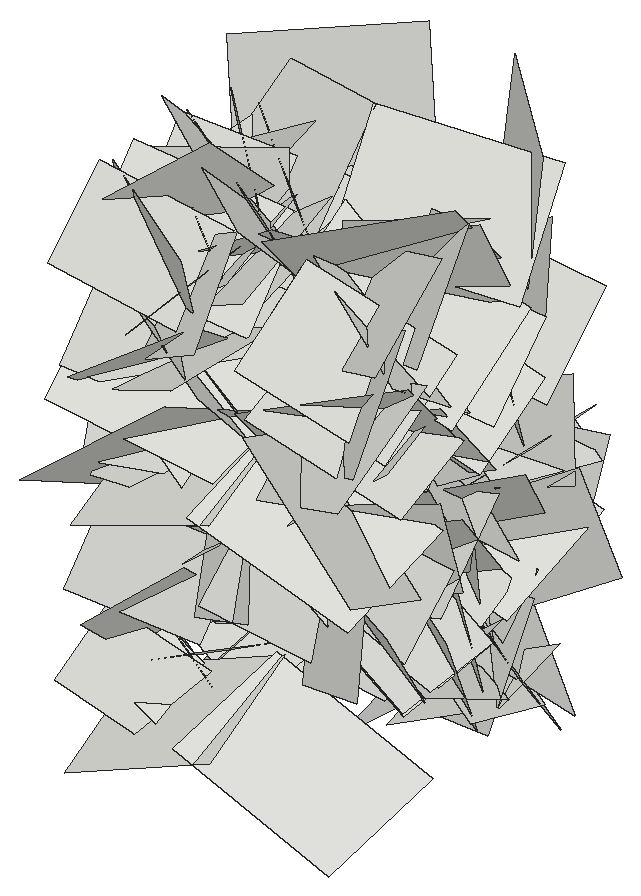
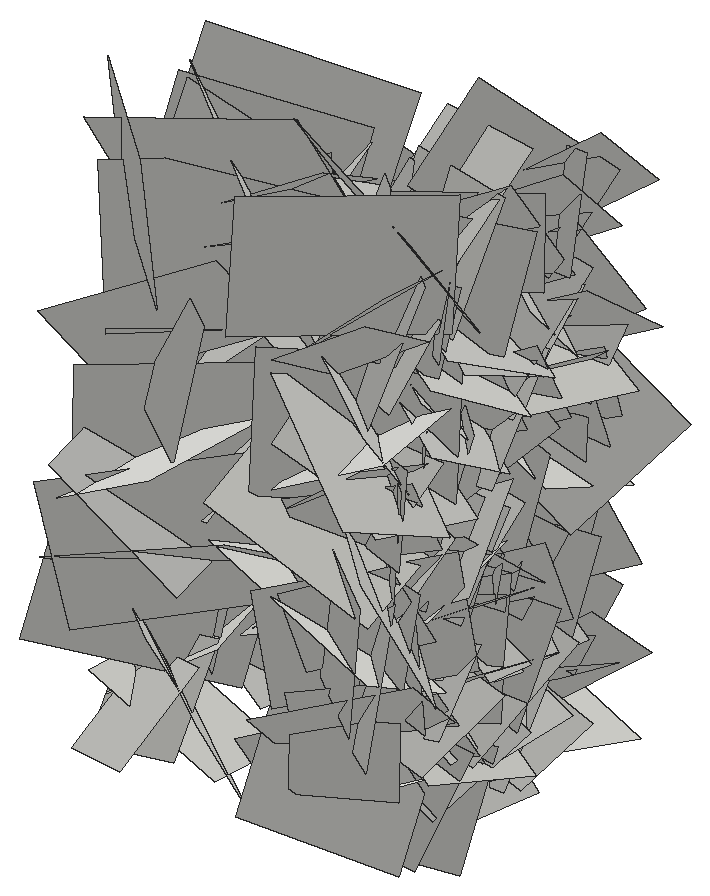
# SketchUp Ruby script. Lengths in inches.
U = 1.inch
M = Sketchup.active_model
def pt(a) = Geom::Point3d.new(a.map { |v| v * U })
def face(e, loops, mat)
  f = e.add_face(loops[0].map { |a| pt(a) })
  loops[1..].each { |l| e.add_face(l.map { |a| pt(a) }).erase! }
  f.material = f.back_material = mat if mat
  f
end
# faces: each face lists its corners as indices into pts; further lists are holes
def faces(e, pts, list, mat = nil) = list.each { |f| face(e, (f[0].is_a?(Array) ? f : [f]).map { |l| l.map { |i| pts[i] } }, mat) }
# xy, xz, yz: faces in a plane at the given z, y or x. An outline is a flat list of corners, or four numbers for a rectangle; further outlines are holes
def ring(l) = l.size == 4 ? [[l[0], l[1]], [l[2], l[1]], [l[2], l[3]], [l[0], l[3]]] : l.each_slice(2).to_a
def flat(e, list, mat, &to3) = list.each { |f| face(e, (f[0].is_a?(Array) ? f : [f]).map { |l| ring(l).map { |u, v| to3.(u, v) } }, mat) }
def xy(e, z, list, mat = nil) = flat(e, list, mat) { |x, y| [x, y, z] }
def xz(e, y, list, mat = nil) = flat(e, list, mat) { |x, z| [x, y, z] }
def yz(e, x, list, mat = nil) = flat(e, list, mat) { |y, z| [x, y, z] }
def lines(e, pts, list) = list.each { |a, b| e.add_line(pt(pts[a]), pt(pts[b])) }
# prism: a flat outline (further loops are holes) pulled along v
def prism(e, loops, v, mat = nil)
  f = face(e, loops, mat); d = Geom::Vector3d.new(v.map { |x| x * U })
  f.pushpull(f.normal.samedirection?(d) ? d.length : -d.length)
end
def box(e, o, s, mat = nil) = prism(e, [[o, [o[0] + s[0], o[1], o[2]], [o[0] + s[0], o[1] + s[1], o[2]], [o[0], o[1] + s[1], o[2]]]], [0, 0, s[2]], mat)
def at(x, y, z, deg = 0) = Geom::Transformation.translation(pt([x, y, z])) * Geom::Transformation.rotation(ORIGIN, Z_AXIS, deg.degrees)
def axes(o, x, y, z) = Geom::Transformation.new([*x, 0, *y, 0, *z, 0, *pt(o).to_a, 1])
def part(name) = M.definitions.add(name)
# library, detail: a bought-in or finely detailed component or shape, given as its bounding box
def library(name, o, s) = part(name).tap { |d| box(d.entities, o, s) }
def detail(e, o, s) = box(e.add_group.entities, o, s)
def put(e, d, t, mat = nil) = e.add_instance(d, t).tap { |i| i.material = mat if mat }
def group(e, t, mat = nil) = e.add_group.tap { |g| g.transformation = t; g.material = mat if mat }.entities
root = M.entities
c1 = part("Component\#6")
p = [[0.01,0,0],[0,3.24,4.54],[4.32,3.24,4.54],[4.33,0,0]]
faces(c1.entities,p,[[0,1,2,3]])
put(root,c1,axes([28.31,163.43,17.5],[0.07736,-0.30856,0.98844],[0.18729,0.98007,0.2929],[-1.08152,0.14765,0.12143]))
put(root,c1,axes([24.34,163.43,17.5],[-0.07736,-0.30856,0.98844],[-0.18729,0.98007,0.2929],[1.08152,0.14765,0.12143]))
put(root,c1,axes([24.34,155.625,2.89],[0.13104,0.56412,0.5606],[-0.11872,0.57403,-0.55293],[0.83462,-0.00692,-0.16667]))
put(root,c1,axes([24.34,168.54,15.47],[-0.051,0.16682,-0.79913],[0.09039,-0.79511,-0.17112],[0.86061,0.0934,-0.02938]))
put(root,c1,axes([28.31,164.44,22.83],[0.02931,-0.02413,-0.88007],[0.04764,-0.87932,0.02552],[-0.93201,-0.0457,-0.02637]))
put(root,c1,axes([24.34,159.9,13.67],[-0.02397,0.44215,0.82689],[-0.11898,0.8199,-0.44149],[0.98679,0.1096,-0.03314]))
put(root,c1,axes([24.34,159.79,6],[-0.13547,0.51146,0.93772],[-0.15367,0.92736,-0.52557],[1.12174,0.18881,0.04125]))
put(root,c1,axes([28.31,165.07,9.38],[-0.13081,0.27606,-0.70722],[0.08788,-0.70731,-0.29057],[-0.79993,-0.12284,0.08373]))
put(root,c1,axes([24.34,167.39,19.82],[0.12929,0.6108,0.35138],[0.02449,0.35295,-0.62154],[0.74654,-0.11736,-0.04046]))
put(root,c1,axes([24.34,155.24,20.59],[0.01301,0.69003,0.71111],[-0.211,0.69839,-0.67424],[1.02891,0.13449,-0.14726]))
put(root,c1,axes([24.34,164.66,7.18],[-0.03191,0.54978,-0.59147],[0.106,-0.58478,-0.54866],[0.84939,0.09364,0.04625]))
put(root,c1,axes([24.34,167.84,10.46],[-0.01526,0.23241,-0.73689],[0.14958,-0.72384,-0.23105],[0.80526,0.13886,0.02896]))
put(root,c1,axes([24.34,166.25,3.34],[0.10377,-0.78092,-0.09398],[-0.04515,-0.09983,0.78516],[0.83253,0.09192,0.05429]))
put(root,c1,axes([24.34,166.67,11.65],[0.03639,0.32382,0.70516],[0.0632,0.70266,-0.32558],[0.82009,-0.06852,-0.0062]))
put(root,c1,axes([28.31,164.7,6.68],[0.19863,-0.78204,0.62344],[0.03401,0.63866,0.7915],[-1.0596,-0.1261,0.14227]))
put(root,c1,axes([28.31,165.06,16.01],[0.24936,0.99659,0.4051],[0.07669,0.39908,-1.02378],[-1.13774,0.24532,0.01978]))
put(root,c1,axes([28.31,162.4,12.14],[-0.15913,-0.1111,0.71617],[0.10617,0.72117,0.13287],[-0.76084,0.12387,-0.13124]))
put(root,c1,axes([24.34,166.02,4.84],[-0.16866,0.71959,0.68076],[0.0323,0.69272,-0.72511],[1.04952,0.09433,0.13172]))
put(root,c1,axes([24.34,157.37,3.29],[0.12325,0.67494,0.21472],[0.06797,0.20667,-0.68436],[0.74769,-0.13004,0.02682]))
put(root,c1,axes([24.34,162.54,0.74],[-0.05881,-0.79857,0.25436],[0.14334,0.24305,0.79255],[0.87675,-0.0933,-0.11251]))
put(root,c1,axes([24.34,164.04,2.37],[-0.08884,-0.86849,0.07962],[0.14736,0.06566,0.86256],[0.91264,-0.09515,-0.13152]))
put(root,c1,axes([28.31,167.12,21.5],[-0.0656,0.35319,-0.61189],[-0.00255,-0.61434,-0.35436],[-0.7489,-0.02885,0.0548]))
put(root,c1,axes([28.31,165.55,15.88],[0.02597,-0.35934,-0.67832],[-0.02345,-0.67872,0.35875],[-0.81334,0.00809,-0.032]))
put(root,c1,axes([28.31,169.26,18.83],[-0.02849,-0.83115,-0.05333],[0.13283,-0.05679,0.82186],[-0.87278,0.01849,0.12683]))
put(root,c1,axes([24.34,168.08,9.41],[-0.11593,0.02752,-0.90523],[0.14705,-0.90054,-0.04413],[0.94866,0.14295,-0.10378]))
put(root,c1,axes([28.31,161.46,7.67],[-0.11157,-0.00104,0.59962],[-0.09459,0.60203,-0.01462],[-0.62852,-0.09042,-0.10424]))
put(root,c1,axes([28.31,169.83,13.22],[-0.13817,-0.64015,-0.16037],[0.03989,-0.17041,0.64965],[-0.69839,0.11692,0.06883]))
put(root,c1,axes([24.34,170.98,12.21],[-0.31631,-0.51758,-1.19288],[-0.16648,-1.20059,0.56021],[1.36826,-0.26573,-0.20761]))
put(root,c1,axes([28.31,164.04,15.7],[-0.03624,-0.6234,-0.24842],[-0.08,-0.24359,0.62167],[-0.70683,0.05954,-0.05762]))
put(root,c1,axes([28.31,160.57,3.12],[-0.03509,0.82869,0.13415],[0.15764,0.13792,-0.81528],[-0.87577,-0.00838,-0.15213]))
put(root,c1,axes([24.34,159.03,23.29],[-0.13252,0.38295,-0.87838],[0.10893,-0.87536,-0.39626],[1.00987,0.14467,-0.07253]))
put(root,c1,axes([28.31,166.8,6.58],[0.19077,-0.84984,-0.315],[-0.00737,-0.32244,0.86593],[-0.9607,-0.16629,-0.0692]))
put(root,c1,axes([24.34,166.22,16.78],[-0.0558,0.90138,-0.08554],[0.09664,-0.07998,-0.89882],[0.95488,0.06076,0.08597]))
put(root,c1,axes([28.31,169.73,5.36],[-0.07377,0.11031,-0.61615],[-0.06228,-0.61836,-0.10407],[-0.66058,0.04598,0.07863]))
put(root,c1,axes([28.31,159.32,12.84],[-0.06752,-0.16321,-0.59207],[-0.0871,-0.58763,0.17083],[-0.64514,0.09641,0.0389]))
put(root,c1,axes([24.34,167.39,3.05],[-0.22625,-1.02118,-0.283],[0.12014,-0.30902,1.02962],[1.11681,-0.17363,-0.16809]))
put(root,c1,axes([28.31,159.79,25.07],[0.1328,0.69586,-0.68383],[0.18687,-0.69425,-0.67416],[-1.01714,-0.03669,-0.21313]))
put(root,c1,axes([24.34,163.26,10.51],[0.09772,0.8385,-0.3881],[-0.10419,-0.37892,-0.842],[0.97385,-0.12468,-0.05114]))
put(root,c1,axes([28.31,160.97,6.7],[-0.04912,0.73058,0.10133],[0.09877,0.10652,-0.72536],[-0.77557,-0.03271,-0.0988]))
put(root,c1,axes([24.34,170.16,13.55],[-0.14984,-1.04824,-0.22204],[0.00627,-0.22472,1.05715],[1.13577,-0.13705,-0.03513]))
put(root,c1,axes([28.31,161.26,10.83],[0.08958,0.45503,-0.59155],[-0.06652,-0.58889,-0.46195],[-0.78829,0.10141,-0.02824]))
put(root,c1,axes([28.31,160.54,14.42],[0.065,-0.29459,-0.75204],[0.0763,-0.74921,0.29935],[-0.85274,-0.0895,-0.03054]))
put(root,c1,axes([28.31,160.65,18.69],[-0.1336,-0.1743,0.59472],[0.06624,0.60023,0.18916],[-0.65357,0.09646,-0.1024]))
put(root,c1,axes([28.31,159.61,12.59],[-0.0897,0.16152,-0.57424],[-0.01993,-0.58042,-0.16049],[-0.632,-0.00462,0.08656]))
put(root,c1,axes([24.34,169.09,13.37],[0.12805,-0.81492,0.2825],[-0.01832,0.28292,0.8235],[0.91406,0.11983,-0.02307]))
put(root,c1,axes([28.31,158.82,19.64],[-0.09205,0.73549,-0.019],[0.17536,0.00088,-0.72213],[-0.75991,-0.08889,-0.16434]))
put(root,c1,axes([24.34,166.72,20.27],[0.14718,0.45385,-0.66356],[0.05291,-0.67695,-0.45256],[0.85051,-0.03642,0.14299]))
put(root,c1,axes([24.34,158.84,13.7],[0.15038,-0.75335,0.50607],[-0.08727,0.49942,0.76653],[0.95804,0.16374,-0.00961]))
put(root,c1,axes([24.34,161.03,4.22],[0.00206,0.54706,-0.73945],[0.10036,-0.73565,-0.544],[0.96983,0.07497,0.05787]))
put(root,c1,axes([24.34,167.74,3.51],[-0.11337,-0.86322,0.3774],[0.28126,0.33685,0.84566],[0.95821,-0.201,-0.20357]))
put(root,c1,axes([24.34,165.75,-1.09],[-0.03685,-0.4153,0.96157],[-0.02645,0.96216,0.41465],[1.10996,0.00914,0.04181]))
put(root,c1,axes([24.34,165.51,17.74],[0.00528,-0.97827,-0.44464],[-0.11526,-0.44282,0.97306],[1.13321,-0.04048,0.10104]))
put(root,c1,axes([28.31,158.25,7.85],[-0.01053,0.60228,-0.51533],[0.19634,-0.49934,-0.58716],[-0.81696,-0.12777,-0.13447]))
put(root,c1,axes([28.31,167.39,12.19],[0.06725,0.11282,-0.6237],[-0.12717,-0.61335,-0.12315],[-0.65971,0.12973,-0.03984]))
put(root,c1,axes([28.31,164.71,11.17],[0.09162,-0.23701,0.75882],[0.09076,0.76162,0.22813],[-0.83777,0.05659,0.1077]))
put(root,c1,axes([24.34,164.72,6.23],[-0.02586,0.29335,1.1723],[-0.23754,1.1511,-0.29271],[1.25874,0.22326,-0.03115]))
put(root,c1,axes([28.31,159.82,10.86],[0.164,0.05549,-0.7166],[-0.119,-0.72215,-0.08015],[-0.75252,0.12629,-0.14349]))
put(root,c1,axes([24.34,167.01,8.33],[0.18631,0.3359,0.73427],[0.04897,0.74605,-0.35235],[0.8545,-0.11599,-0.1399]))
put(root,c1,axes([24.34,166.18,19.56],[-0.12535,0.0531,1.28965],[-0.2192,1.27754,-0.07157],[1.35051,0.21229,0.10808]))
put(root,c1,axes([24.34,168.14,0.12],[-0.06773,-0.63363,0.78179],[0.11595,0.77435,0.63654],[1.06038,-0.12515,-0.01967]))
put(root,c1,axes([24.34,169.19,10.7],[-0.0913,0.46499,-1.24639],[-0.29576,-1.22753,-0.43867],[1.37875,-0.23253,-0.17663]))
put(root,c1,axes([28.31,165.96,10.85],[0.09912,0.20412,-0.70693],[0.02587,-0.71308,-0.20267],[-0.77953,0.00229,-0.09661]))
put(root,c1,axes([28.31,161.25,17.66],[0.25985,0.898,-0.37026],[0.14737,-0.41038,-0.90325],[-1.01902,0.16964,-0.22504]))
put(root,c1,axes([28.31,162.79,15.86],[0.07285,0.46729,0.4905],[-0.02436,0.49435,-0.46773],[-0.71769,0.03066,0.06566]))
put(root,c1,axes([24.34,167.22,15.375],[-0.0235,-0.92066,-0.53568],[-0.01768,-0.53543,0.92093],[1.12894,-0.02755,0.00327]))
put(root,c1,axes([24.34,167.28,17.92],[-0.19972,-0.96368,-0.57877],[0.14667,-0.60226,0.95775],[1.18251,-0.08806,-0.21655]))
put(root,c1,axes([24.34,157.18,19.73],[-0.07599,0.81527,0.8297],[-0.084,0.82592,-0.8184],[1.23014,0.10676,-0.00463]))
put(root,c1,axes([24.34,167.18,1.59],[-0.07507,-1.0991,0.32301],[-0.05871,0.32653,1.09895],[1.2129,-0.05222,0.07319]))
put(root,c1,axes([24.34,168.87,14.79],[0.03205,0.06087,-1.12787],[-0.16204,-1.11767,-0.06442],[1.18627,-0.15431,0.02167]))
put(root,c1,axes([24.34,166.01,11.8],[0.21466,0.53877,-0.68228],[-0.03009,-0.69607,-0.55809],[0.92102,-0.14831,0.14079]))
put(root,c1,axes([24.34,163.57,3.71],[0.11292,-0.2033,0.99476],[-0.09749,0.99417,0.21302],[1.07181,0.11185,-0.08542]))
put(root,c1,axes([24.34,159.91,9.22],[-0.2022,-1.20502,0.50539],[-0.1049,0.52261,1.20871],[1.38114,-0.13672,0.1658]))
put(root,c1,axes([24.34,162.44,14.8125],[-0.22172,-1.13603,-0.19278],[0.19013,-0.22565,1.13507],[1.20652,-0.17321,-0.21429]))
put(root,c1,axes([24.34,160.62,5.12],[0.08568,1.04485,0.18773],[-0.09569,0.19436,-1.04286],[1.1212,-0.06325,-0.10335]))
put(root,c1,axes([28.31,162.91,7.6875],[0.03517,0.6334,0.29771],[0.1292,0.28826,-0.62688],[-0.73053,0.08147,-0.09654]))
put(root,c1,axes([24.34,163.93,5.47],[0.11462,-1.01834,-0.26907],[-0.10191,-0.2789,1.0169],[1.11183,0.07941,0.12095]))
put(root,c1,axes([24.34,156.14,6.5],[0.17845,0.35117,0.84391],[0.01887,0.85668,-0.36003],[0.96872,-0.08137,-0.14844]))
put(root,c1,axes([28.31,170.02,6.34],[0.13634,-0.30577,-0.6303],[0.02329,-0.63876,0.31436],[-0.74222,-0.07621,-0.10592]))
put(root,c1,axes([24.34,160.14,4.78],[0.03826,-0.47304,0.81506],[0.18962,0.80427,0.45886],[0.98077,-0.13704,-0.12051]))
put(root,c1,axes([24.34,166.625,12.7],[0.17127,1.04033,-0.10676],[-0.13463,-0.08771,-1.04688],[1.10034,-0.17266,-0.11147]))
put(root,c1,axes([24.34,168.99,0.33],[0.20008,-0.71049,0.66963],[-0.07161,0.67089,0.73087],[1.03242,0.18422,-0.07908]))
put(root,c1,axes([24.34,164.18,5.53],[0.00871,-1.21515,-0.1589],[-0.11926,-0.15898,1.20995],[1.29354,-0.00648,0.11262]))
put(root,c1,axes([28.31,159.77,13.93],[0.14822,0.47929,0.38572],[-0.01533,0.39801,-0.48932],[-0.65196,0.0996,0.0992]))
put(root,c1,axes([24.34,165.6875,8.33],[0.14254,-0.77018,0.64298],[0.05856,0.65343,0.77114],[1.06187,0.06735,-0.12884]))
put(root,c1,axes([24.34,164.53,2.65],[0.11418,0.95876,0.15487],[0.16789,0.13639,-0.95453],[1.01568,-0.13033,0.14037]))
put(root,c1,axes([24.34,170.79,17.67],[0.07972,-0.69903,-0.88266],[-0.01234,-0.88506,0.69994],[1.19343,0.03754,0.0662]))
put(root,c1,axes([24.34,165.97,13.03],[0.11695,-0.23373,1.15092],[-0.10796,1.14973,0.24325],[1.24018,0.12213,-0.08736]))
put(root,c1,axes([28.31,164.09,3.1],[0.16189,-0.51758,0.36968],[0.06161,0.38995,0.52196],[-0.67139,-0.08902,0.13704]))
put(root,c1,axes([24.34,155.93,16.01],[0.06166,0.77521,1.08886],[-0.24821,1.07895,-0.75564],[1.39492,0.15772,-0.18259]))
put(root,c1,axes([24.34,163.21,2.24],[-0.08398,-0.53221,1.10764],[0.11648,1.10243,0.53756],[1.29738,-0.13342,0.02343]))
put(root,c1,axes([24.34,161.02,12.77],[0.04866,0.36936,-1.04237],[0.12613,-1.03886,-0.36288],[1.16543,0.09701,0.0828]))
put(root,c1,axes([24.34,162.03,18.62],[0.15865,-0.78055,-0.79386],[-0.03617,-0.80384,0.78393],[1.17956,0.08034,0.13081]))
put(root,c1,axes([24.34,161.03,16.77],[-0.02327,0.73455,-0.90907],[0.17416,-0.89826,-0.72978],[1.22657,0.14148,0.08637]))
put(root,c1,axes([24.34,163.86,1.73],[0.03729,0.66749,1.03354],[-0.00972,1.03407,-0.66752],[1.30413,-0.01138,-0.03452]))
put(root,c1,axes([24.34,162.85,15.75],[0.04254,-1.00522,0.67204],[0.02385,0.67292,1.00519],[1.28151,0.02084,-0.04102]))
put(root,c1,axes([24.34,163.36,23.49],[0.04873,0.57368,-1.00395],[0.12423,-1.00188,-0.56714],[1.21936,0.07915,0.09791]))
put(root,c1,axes([24.34,159.69,18.96],[0.02704,0.74145,1.09535],[-0.09362,1.09406,-0.73853],[1.39894,0.05888,-0.07059]))
put(root,c1,axes([24.34,166.4,18.65],[-0.092,-1.19571,-0.63762],[0.0325,-0.6405,1.19693],[1.43603,-0.06211,-0.06794]))
put(root,c1,axes([24.34,155.03,14.95],[-0.10989,1.07322,0.82249],[0.07177,0.82799,-1.07186],[1.43147,0.04087,0.11688]))
put(root,c1,axes([24.34,159.14,18.38],[0.07521,0.79304,-0.86536],[0.12573,-0.86735,-0.78513],[1.23784,0.03991,0.13233]))
put(root,c1,axes([24.34,168.375,23.9],[-0.0952,-0.72561,-1.04974],[0.29336,-1.03837,0.69407],[1.32049,0.17837,-0.22987]))
put(root,c1,axes([24.34,157.93,15.34],[0.27083,1.19165,0.15594],[-0.0802,0.17506,-1.21378],[1.27139,-0.2428,-0.10978]))
put(root,c1,axes([24.34,162.31,11.53],[0.17206,0.75955,-0.87532],[0.12131,-0.89005,-0.75111],[1.22246,-0.01858,0.19774]))
put(root,c1,axes([24.34,165.1,2.71],[-0.06092,-1.21711,0.58199],[0.18306,0.57109,1.21136],[1.41828,-0.12599,-0.13136]))
put(root,c1,axes([24.34,170.58,10.37],[0.24309,-1.14649,0.14454],[0.04952,0.15643,1.16674],[1.2239,0.22139,-0.07591]))
put(root,c1,axes([24.34,161.07,7.88],[0.0926,0.91308,0.78861],[0.24837,0.76278,-0.90913],[1.25453,-0.21841,0.12178]))
put(root,c1,axes([24.34,171.01,11.29],[0.23144,-0.15428,-1.27652],[-0.01824,-1.29503,0.15357],[1.36284,0.00887,0.21884]))
put(root,c1,axes([24.34,167.61,21.95],[0.32344,0.31012,-1.26322],[-0.1451,-1.28265,-0.34796],[1.37111,-0.2089,0.26116]))
put(root,c1,axes([24.34,161.91,24.73],[0.20116,0.87735,-0.9177],[0.06395,-0.93308,-0.87958],[1.34427,-0.0869,0.17917]))
put(root,c1,axes([24.34,161.24,11.55],[0.08722,-1.18104,-0.51149],[0.30261,-0.48302,1.16122],[1.33028,0.18731,-0.23062]))
put(root,c1,axes([24.34,160.65,1.35],[0.1594,-1.22011,-0.46707],[0.28659,-0.43091,1.2127],[1.35486,0.2347,-0.20157]))
put(root,c1,axes([24.34,170.67,8.29],[0.13658,-1.14766,-0.62909],[0.33753,-0.58565,1.13362],[1.34561,0.26339,-0.2205]))
put(root,c1,axes([24.34,161.87,9.58],[0.35888,-0.49511,-1.17449],[0.11741,-1.19919,0.53746],[1.34594,0.23663,0.26628]))
put(root,c1,axes([38.11,161.87,9.58],[-0.35888,-0.49511,-1.17449],[-0.11741,-1.19919,0.53746],[-1.34594,0.23663,0.26628]))
put(root,c1,axes([38.11,170.67,8.29],[-0.13658,-1.14766,-0.62909],[-0.33753,-0.58565,1.13362],[-1.34561,0.26339,-0.2205]))
put(root,c1,axes([38.11,160.65,1.35],[-0.1594,-1.22011,-0.46707],[-0.28659,-0.43091,1.2127],[-1.35486,0.2347,-0.20157]))
put(root,c1,axes([38.11,161.24,11.55],[-0.08722,-1.18104,-0.51149],[-0.30261,-0.48302,1.16122],[-1.33028,0.18731,-0.23062]))
put(root,c1,axes([38.11,161.91,24.73],[-0.20116,0.87735,-0.9177],[-0.06395,-0.93308,-0.87958],[-1.34427,-0.0869,0.17917]))
put(root,c1,axes([38.11,167.61,21.95],[-0.32344,0.31012,-1.26322],[0.1451,-1.28265,-0.34796],[-1.37111,-0.2089,0.26116]))
put(root,c1,axes([38.11,171.01,11.29],[-0.23144,-0.15428,-1.27652],[0.01824,-1.29503,0.15357],[-1.36284,0.00887,0.21884]))
put(root,c1,axes([38.11,161.07,7.88],[-0.0926,0.91308,0.78861],[-0.24837,0.76278,-0.90913],[-1.25453,-0.21841,0.12178]))
put(root,c1,axes([38.11,170.58,10.37],[-0.24309,-1.14649,0.14454],[-0.04952,0.15643,1.16674],[-1.2239,0.22139,-0.07591]))
put(root,c1,axes([38.11,165.1,2.71],[0.06092,-1.21711,0.58199],[-0.18306,0.57109,1.21136],[-1.41828,-0.12599,-0.13136]))
put(root,c1,axes([38.11,162.31,11.53],[-0.17206,0.75955,-0.87532],[-0.12131,-0.89005,-0.75111],[-1.22246,-0.01858,0.19774]))
put(root,c1,axes([38.11,157.93,15.34],[-0.27083,1.19165,0.15594],[0.0802,0.17506,-1.21378],[-1.27139,-0.2428,-0.10978]))
put(root,c1,axes([38.11,168.375,23.9],[0.0952,-0.72561,-1.04974],[-0.29336,-1.03837,0.69407],[-1.32049,0.17837,-0.22987]))
put(root,c1,axes([38.11,159.14,18.38],[-0.07521,0.79304,-0.86536],[-0.12573,-0.86735,-0.78513],[-1.23784,0.03991,0.13233]))
put(root,c1,axes([38.11,155.03,14.95],[0.10989,1.07322,0.82249],[-0.07177,0.82799,-1.07186],[-1.43147,0.04087,0.11688]))
put(root,c1,axes([38.11,166.4,18.65],[0.092,-1.19571,-0.63762],[-0.0325,-0.6405,1.19693],[-1.43603,-0.06211,-0.06794]))
put(root,c1,axes([38.11,159.69,18.96],[-0.02704,0.74145,1.09535],[0.09362,1.09406,-0.73853],[-1.39894,0.05888,-0.07059]))
put(root,c1,axes([38.11,163.36,23.49],[-0.04873,0.57368,-1.00395],[-0.12423,-1.00188,-0.56714],[-1.21936,0.07915,0.09791]))
put(root,c1,axes([38.11,162.85,15.75],[-0.04254,-1.00522,0.67204],[-0.02385,0.67292,1.00519],[-1.28151,0.02084,-0.04102]))
put(root,c1,axes([38.11,163.86,1.73],[-0.03729,0.66749,1.03354],[0.00972,1.03407,-0.66752],[-1.30413,-0.01138,-0.03452]))
put(root,c1,axes([38.11,161.03,16.77],[0.02327,0.73455,-0.90907],[-0.17416,-0.89826,-0.72978],[-1.22657,0.14148,0.08637]))
put(root,c1,axes([38.11,162.03,18.62],[-0.15865,-0.78055,-0.79386],[0.03617,-0.80384,0.78393],[-1.17956,0.08034,0.13081]))
put(root,c1,axes([38.11,161.02,12.77],[-0.04866,0.36936,-1.04237],[-0.12613,-1.03886,-0.36288],[-1.16543,0.09701,0.0828]))
put(root,c1,axes([38.11,163.21,2.24],[0.08398,-0.53221,1.10764],[-0.11648,1.10243,0.53756],[-1.29738,-0.13342,0.02343]))
put(root,c1,axes([38.11,155.93,16.01],[-0.06166,0.77521,1.08886],[0.24821,1.07895,-0.75564],[-1.39492,0.15772,-0.18259]))
put(root,c1,axes([34.14,164.09,3.1],[-0.16189,-0.51758,0.36968],[-0.06161,0.38995,0.52196],[0.67139,-0.08902,0.13704]))
put(root,c1,axes([38.11,165.97,13.03],[-0.11695,-0.23373,1.15092],[0.10796,1.14973,0.24325],[-1.24018,0.12213,-0.08736]))
put(root,c1,axes([38.11,170.79,17.67],[-0.07972,-0.69903,-0.88266],[0.01234,-0.88506,0.69994],[-1.19343,0.03754,0.0662]))
put(root,c1,axes([38.11,164.53,2.65],[-0.11418,0.95876,0.15487],[-0.16789,0.13639,-0.95453],[-1.01568,-0.13033,0.14037]))
put(root,c1,axes([38.11,165.6875,8.33],[-0.14254,-0.77018,0.64298],[-0.05856,0.65343,0.77114],[-1.06187,0.06735,-0.12884]))
put(root,c1,axes([34.14,159.77,13.93],[-0.14822,0.47929,0.38572],[0.01533,0.39801,-0.48932],[0.65196,0.0996,0.0992]))
put(root,c1,axes([38.11,164.18,5.53],[-0.00871,-1.21515,-0.1589],[0.11926,-0.15898,1.20995],[-1.29354,-0.00648,0.11262]))
put(root,c1,axes([38.11,168.99,0.33],[-0.20008,-0.71049,0.66963],[0.07161,0.67089,0.73087],[-1.03242,0.18422,-0.07908]))
put(root,c1,axes([38.11,166.625,12.7],[-0.17127,1.04033,-0.10676],[0.13463,-0.08771,-1.04688],[-1.10034,-0.17266,-0.11147]))
put(root,c1,axes([38.11,160.14,4.78],[-0.03826,-0.47304,0.81506],[-0.18962,0.80427,0.45886],[-0.98077,-0.13704,-0.12051]))
put(root,c1,axes([34.14,170.02,6.34],[-0.13634,-0.30577,-0.6303],[-0.02329,-0.63876,0.31436],[0.74222,-0.07621,-0.10592]))
put(root,c1,axes([38.11,156.14,6.5],[-0.17845,0.35117,0.84391],[-0.01887,0.85668,-0.36003],[-0.96872,-0.08137,-0.14844]))
put(root,c1,axes([38.11,163.93,5.47],[-0.11462,-1.01834,-0.26907],[0.10191,-0.2789,1.0169],[-1.11183,0.07941,0.12095]))
put(root,c1,axes([34.14,162.91,7.6875],[-0.03517,0.6334,0.29771],[-0.1292,0.28826,-0.62688],[0.73053,0.08147,-0.09654]))
put(root,c1,axes([38.11,160.62,5.12],[-0.08568,1.04485,0.18773],[0.09569,0.19436,-1.04286],[-1.1212,-0.06325,-0.10335]))
put(root,c1,axes([38.11,162.44,14.8125],[0.22172,-1.13603,-0.19278],[-0.19013,-0.22565,1.13507],[-1.20652,-0.17321,-0.21429]))
put(root,c1,axes([38.11,159.91,9.22],[0.2022,-1.20502,0.50539],[0.1049,0.52261,1.20871],[-1.38114,-0.13672,0.1658]))
put(root,c1,axes([38.11,163.57,3.71],[-0.11292,-0.2033,0.99476],[0.09749,0.99417,0.21302],[-1.07181,0.11185,-0.08542]))
put(root,c1,axes([38.11,166.01,11.8],[-0.21466,0.53877,-0.68228],[0.03009,-0.69607,-0.55809],[-0.92102,-0.14831,0.14079]))
put(root,c1,axes([38.11,168.87,14.79],[-0.03205,0.06087,-1.12787],[0.16204,-1.11767,-0.06442],[-1.18627,-0.15431,0.02167]))
put(root,c1,axes([38.11,167.18,1.59],[0.07507,-1.0991,0.32301],[0.05871,0.32653,1.09895],[-1.2129,-0.05222,0.07319]))
put(root,c1,axes([38.11,157.18,19.73],[0.07599,0.81527,0.8297],[0.084,0.82592,-0.8184],[-1.23014,0.10676,-0.00463]))
put(root,c1,axes([38.11,167.28,17.92],[0.19972,-0.96368,-0.57877],[-0.14667,-0.60226,0.95775],[-1.18251,-0.08806,-0.21655]))
put(root,c1,axes([38.11,167.22,15.375],[0.0235,-0.92066,-0.53568],[0.01768,-0.53543,0.92093],[-1.12894,-0.02755,0.00327]))
put(root,c1,axes([34.14,162.79,15.86],[-0.07285,0.46729,0.4905],[0.02436,0.49435,-0.46773],[0.71769,0.03066,0.06566]))
put(root,c1,axes([34.14,161.25,17.66],[-0.25985,0.898,-0.37026],[-0.14737,-0.41038,-0.90325],[1.01902,0.16964,-0.22504]))
put(root,c1,axes([34.14,165.96,10.85],[-0.09912,0.20412,-0.70693],[-0.02587,-0.71308,-0.20267],[0.77953,0.00229,-0.09661]))
put(root,c1,axes([38.11,169.19,10.7],[0.0913,0.46499,-1.24639],[0.29576,-1.22753,-0.43867],[-1.37875,-0.23253,-0.17663]))
put(root,c1,axes([38.11,168.14,0.12],[0.06773,-0.63363,0.78179],[-0.11595,0.77435,0.63654],[-1.06038,-0.12515,-0.01967]))
put(root,c1,axes([38.11,166.18,19.56],[0.12535,0.0531,1.28965],[0.2192,1.27754,-0.07157],[-1.35051,0.21229,0.10808]))
